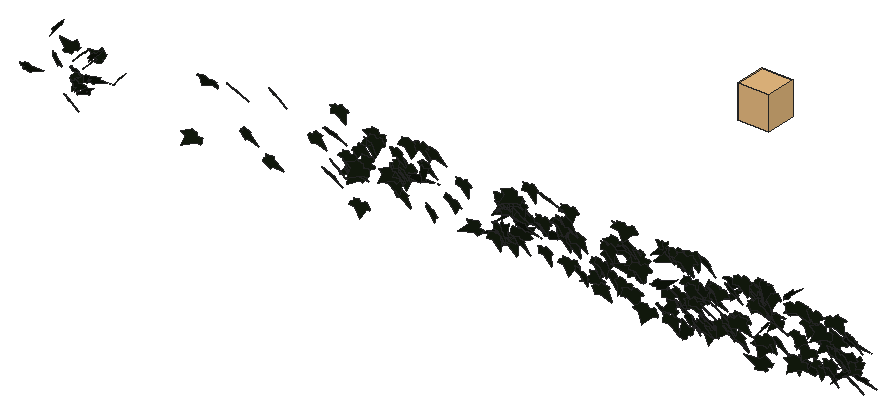
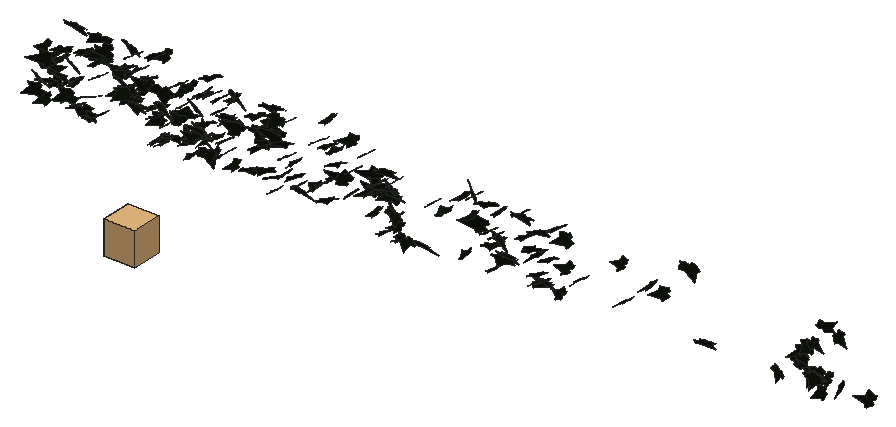
# SketchUp Ruby script. Lengths in millimetres.
U = 1.mm
M = Sketchup.active_model
def pt(a) = Geom::Point3d.new(a.map { |v| v * U })
def face(e, loops, mat)
  f = e.add_face(loops[0].map { |a| pt(a) })
  loops[1..].each { |l| e.add_face(l.map { |a| pt(a) }).erase! }
  f.material = f.back_material = mat if mat
  f
end
# faces: each face lists its corners as indices into pts; further lists are holes
def faces(e, pts, list, mat = nil) = list.each { |f| face(e, (f[0].is_a?(Array) ? f : [f]).map { |l| l.map { |i| pts[i] } }, mat) }
# xy, xz, yz: faces in a plane at the given z, y or x. An outline is a flat list of corners, or four numbers for a rectangle; further outlines are holes
def ring(l) = l.size == 4 ? [[l[0], l[1]], [l[2], l[1]], [l[2], l[3]], [l[0], l[3]]] : l.each_slice(2).to_a
def flat(e, list, mat, &to3) = list.each { |f| face(e, (f[0].is_a?(Array) ? f : [f]).map { |l| ring(l).map { |u, v| to3.(u, v) } }, mat) }
def xy(e, z, list, mat = nil) = flat(e, list, mat) { |x, y| [x, y, z] }
def xz(e, y, list, mat = nil) = flat(e, list, mat) { |x, z| [x, y, z] }
def yz(e, x, list, mat = nil) = flat(e, list, mat) { |y, z| [x, y, z] }
def lines(e, pts, list) = list.each { |a, b| e.add_line(pt(pts[a]), pt(pts[b])) }
# prism: a flat outline (further loops are holes) pulled along v
def prism(e, loops, v, mat = nil)
  f = face(e, loops, mat); d = Geom::Vector3d.new(v.map { |x| x * U })
  f.pushpull(f.normal.samedirection?(d) ? d.length : -d.length)
end
def box(e, o, s, mat = nil) = prism(e, [[o, [o[0] + s[0], o[1], o[2]], [o[0] + s[0], o[1] + s[1], o[2]], [o[0], o[1] + s[1], o[2]]]], [0, 0, s[2]], mat)
def at(x, y, z, deg = 0) = Geom::Transformation.translation(pt([x, y, z])) * Geom::Transformation.rotation(ORIGIN, Z_AXIS, deg.degrees)
def axes(o, x, y, z) = Geom::Transformation.new([*x, 0, *y, 0, *z, 0, *pt(o).to_a, 1])
def part(name) = M.definitions.add(name)
# library, detail: a bought-in or finely detailed component or shape, given as its bounding box
def library(name, o, s) = part(name).tap { |d| box(d.entities, o, s) }
def detail(e, o, s) = box(e.add_group.entities, o, s)
def put(e, d, t, mat = nil) = e.add_instance(d, t).tap { |i| i.material = mat if mat }
def group(e, t, mat = nil) = e.add_group.tap { |g| g.transformation = t; g.material = mat if mat }.entities
root = M.entities
M.materials.add("efeu1").color = [18, 25, 13]
c1 = part("ivyleaf_9")
p = [[39.1,54.8,31.7],[34.5,51.8,30.2],[-5.3,25.2,17.3],[-17.9,28.3,20.9],[-21.6,21.7,17],[-20.2,4.3,5.3],
  [-22.9,-0.3,2.5],[-17.1,-4,-0.6],[-2,-2.1,-1.2],[-0.7,-15.4,-10.1],[16.6,-22.3,-16.7],[21.1,-15.1,-12.5],
  [32.7,-10.7,-11],[46.1,-1.8,-6.6],[30.8,11.2,3.8]]
faces(c1.entities,p,[[0,1,2,3,4,5,6,7,8,9,10,11,12,13,14]],"efeu1")
c2 = library("Spot Light\#3",[-129.6,-129.6,-280.7],[259.2,259.2,280.7])
put(root,c1,axes([27.4,438.3,4934.8],[1.05185,-0.2815,1.21489],[1.46396,-0.21485,-0.90136],[0.41422,1.47415,0.10062]))
put(root,c1,axes([196.1,533.2,5034.4],[1.27663,-0.50201,-0.87336],[-0.8789,0.50729,-1.15475],[0.85903,1.26507,0.11648]))
put(root,c1,axes([300.8,452.1,5346.7],[-0.65532,1.10379,-0.87415],[0.38789,-0.81635,-1.22618],[-1.6734,-0.62148,0.0581]))
put(root,c1,axes([317.8,578.5,4960.4],[1.59905,-0.3934,0.25738],[0.29827,-0.08077,-1.36844],[0.48988,1.33329,-0.00695]))
put(root,c1,axes([454.3,467,4996.8],[-1.46158,-0.32954,-0.68957],[0.90027,-0.16502,-1.20316],[0.2427,-1.37241,0.31025]))
put(root,c1,axes([463.1,479,4983.5],[0.96181,1.16892,0.14934],[0.09715,0.12643,-1.40993],[-1.43439,0.79237,0.00465]))
put(root,c1,axes([507.7,343.1,5276],[0.22927,0.30059,1.46884],[-1.80845,0.25923,0.1366],[-0.27428,-1.45795,0.32713]))
put(root,c1,axes([463,333.7,4901.5],[1.4272,-0.88217,0.28166],[0.28289,-0.16031,-1.46513],[1.09379,1.19254,0.01141]))
put(root,c1,axes([509,407.6,4987.3],[0.93054,0.60119,-1.10895],[-1.1764,-0.55762,-0.96552],[-0.99218,1.22499,0.10473]))
put(root,c1,axes([520.2,565.9,5150.3],[-0.19925,1.30316,-0.58109],[-0.04644,-0.58866,-1.30942],[-1.74013,-0.13351,0.10148]))
put(root,c1,axes([526.5,442.4,5215.2],[-0.8899,1.02361,-0.70913],[0.05509,-0.79955,-1.20058],[-1.51821,-0.629,0.37209]))
put(root,c1,axes([547.3,595.1,5113.7],[-0.56172,0.32471,1.30651],[-1.30957,0.74482,-0.56339],[-0.99127,-1.16799,0.00394]))
put(root,c1,axes([538.7,403.6,4944.4],[0.97215,1.17437,0.25341],[0.14251,0.2269,-1.41887],[-1.45876,0.80479,0.03026]))
put(root,c1,axes([576.3,410.4,5146.4],[0.66606,0.90484,1.05669],[0.25898,1.06766,-1.02392],[-1.67733,0.52415,0.26151]))
put(root,c1,axes([630.5,393.8,5064.3],[1.44137,0.239,0.91451],[1.06503,0.28542,-1.20239],[-0.44218,1.46653,0.08497]))
put(root,c1,axes([694.7,586.7,4995.8],[0.16272,1.21568,0.7693],[-0.05802,0.7759,-1.21787],[-1.75419,0.0871,0.11164]))
put(root,c1,axes([1454.1,460.6,4897.8],[-2.30508,-0.52096,0.19612],[-0.36198,-0.05406,-1.31821],[0.99566,-1.22574,-0.02521]))
put(root,c1,axes([1591.9,413.9,5400.5],[1.5052,0.38712,-1.07511],[-1.91846,-0.37942,-0.87815],[-1.02421,1.2796,0.06487]))
put(root,c1,axes([1620.8,619.3,5265.3],[2.08359,-0.78677,0.26516],[0.48322,-0.10053,-1.34658],[1.50443,1.12194,0.06528]))
put(root,c1,axes([1921.4,392.3,5129.5],[1.44859,-1.06438,-0.49172],[-0.30778,0.48534,-1.30088],[2.21012,0.76522,0.14113]))
put(root,c1,axes([1991.3,606.3,5352.2],[1.37791,-1.03353,0.55169],[0.52453,-0.48009,-1.26106],[2.16713,0.77334,-0.04555]))
put(root,c1,axes([2093.1,420.9,4969.4],[1.52697,-0.79111,-0.80628],[-0.37249,0.87665,-1.05491],[2.1173,0.72477,0.39589]))
put(root,c1,axes([2322.6,627.4,5138.8],[0.76828,-1.09674,-0.68829],[-0.14175,0.7001,-1.15924],[2.46024,0.38282,0.14815]))
put(root,c1,axes([2489.8,642.5,4960.6],[0.75382,-0.95937,0.84674],[0.61245,-0.78321,-1.03792],[2.35706,0.51033,-0.00111]))
put(root,c1,axes([2549.8,599.7,5437.9],[0.01755,-1.33902,-0.38342],[0.03213,0.38351,-1.33892],[2.65065,0.00421,0.01877]))
put(root,c1,axes([2534.6,505.5,5303.9],[2.46874,-0.55053,0.23449],[0.40086,-0.1039,-1.40908],[1.06596,1.31407,-0.01317]))
put(root,c1,axes([2587.1,442.8,5031.7],[1.09046,-1.14178,0.59781],[0.78836,-0.45636,-1.26865],[2.32272,0.69093,0.14994]))
put(root,c1,axes([2668.2,641.4,5011.9],[-2.56331,-0.00456,0.09388],[-0.17862,-0.00694,-1.34683],[0.00958,-1.35009,0.00661]))
put(root,c1,axes([2685.2,634.8,4969.2],[-1.39839,-1.00394,0.51386],[-0.5806,-0.41352,-1.24409],[2.06644,-0.79557,-0.00181]))
put(root,c1,axes([2649.2,634.7,5013.6],[0.60769,-1.07225,-0.76696],[0.3,0.81452,-1.07313],[2.49102,0.16349,0.31634]))
put(root,c1,axes([2675.7,567.9,5134.7],[-0.94128,-1.26783,0.04544],[-0.01331,-0.04605,-1.36085],[2.41445,-0.49452,0.01022]))
put(root,c1,axes([2708.9,611,5186.2],[0.81813,-0.73139,-1.07949],[-0.45428,1.0733,-0.82225],[2.43971,0.44511,0.20889]))
put(root,c1,axes([2853.7,556.1,5138.9],[-1.39855,-0.28673,1.11502],[-1.8365,-0.56812,-0.78203],[1.19515,-1.20851,0.10308]))
put(root,c1,axes([2830.1,608.1,5275.6],[-0.51347,-1.3436,-0.18841],[0.02425,0.18958,-1.3702],[2.58204,-0.26897,-0.0246]))
put(root,c1,axes([2872.4,435.9,4898.2],[-0.87636,-1.26984,-0.02353],[-0.01503,0.02789,-1.35064],[2.41712,-0.46022,-0.01693]))
put(root,c1,axes([2904.4,402.6,5191.3],[-2.02144,-0.92998,0.44622],[-0.58815,-0.32417,-1.4112],[1.87296,-1.1055,0.03845]))
put(root,c1,axes([2914.8,560.2,5383],[-2.49156,-0.45963,-0.17804],[0.30501,0.08089,-1.38729],[0.88713,-1.31872,-0.02305]))
put(root,c1,axes([2937.6,517.9,5369.9],[-0.40079,-1.3596,0.21791],[-0.11885,-0.21078,-1.3755],[2.61792,-0.21772,-0.02909]))
put(root,c1,axes([3000.1,617.9,5083.2],[-2.58496,-0.18615,0.01166],[-0.00965,-0.04877,-1.37009],[0.35484,-1.35739,0.04763]))
put(root,c1,axes([3002.3,615.5,5051.4],[-1.51928,-0.58379,-0.95076],[1.4529,0.56673,-0.98896],[1.54848,-1.10454,-0.00491]))
put(root,c1,axes([3063.2,601.3,5191.8],[-0.82913,1.30172,0.21151],[-0.1436,0.19778,-1.37266],[-2.50581,-0.44205,0.00868]))
put(root,c1,axes([3029.9,607.7,5155.3],[0.79861,-1.30874,0.10938],[0.04056,-0.10802,-1.37431],[2.49915,0.41996,-0.01265]))
put(root,c1,axes([3050.7,625.1,4964.6],[0.76216,-1.2942,-0.11492],[0.14171,0.14291,-1.35003],[2.46876,0.39135,0.11297]))
put(root,c1,axes([3067.2,604.7,5198],[0.28453,-1.3587,-0.23646],[-0.00235,0.23772,-1.36669],[2.62475,0.1475,0.02441]))
put(root,c1,axes([3107.6,611.9,5120.5],[-1.01144,-1.22449,-0.33365],[0.1904,0.32018,-1.3344],[2.4079,-0.53966,-0.03464]))
put(root,c1,axes([3090.7,529.2,5335.7],[0.94962,-1.29655,-0.07612],[-0.03525,0.07443,-1.38921],[2.47158,0.49921,0.00943]))
put(root,c1,axes([3135.9,604,5204.8],[-0.34265,-1.37168,0.08],[0.01061,-0.08141,-1.38335],[2.61499,-0.1794,0.01609]))
put(root,c1,axes([3172.3,591.3,5398.3],[-1.26405,-1.19263,-0.35048],[0.56016,0.23519,-1.35808],[2.29853,-0.71319,0.13823]))
put(root,c1,axes([3235.2,539.9,5179.2],[1.75515,-0.22884,1.07308],[2.06405,-0.02249,-0.93683],[0.31672,1.41473,0.15868]))
put(root,c1,axes([3269.2,579.1,5416.7],[0.42641,-1.38648,-0.15003],[0.03127,0.15456,-1.40388],[2.65397,0.22094,0.04064]))
put(root,c1,axes([3270.7,596.1,5270.7],[1.39207,-1.16552,-0.24444],[-0.01661,0.28161,-1.36887],[2.26642,0.71794,0.14011]))
put(root,c1,axes([3338.9,593.4,4944.2],[0.21321,-1.0973,0.79828],[0.13508,-0.79516,-1.10297],[2.57901,0.13236,-0.00822]))
put(root,c1,axes([3343.1,586.3,5393],[1.50238,-1.09313,-0.41091],[-0.02661,0.4871,-1.32267],[2.22241,0.7448,0.26195]))
put(root,c1,axes([3389.8,435.3,5286.3],[-0.32853,0.80836,1.24038],[0.05217,-1.24682,0.81637],[2.81727,0.11735,0.12953]))
put(root,c1,axes([3588.2,510.7,5142.5],[-0.24682,-1.22769,0.81297],[0.46358,-0.82276,-1.20362],[2.76378,0.02836,0.27449]))
put(root,c1,axes([3608.9,596.2,5251.1],[0.18815,-1.39101,0.07323],[-0.0011,-0.07346,-1.3945],[2.65103,0.09869,-0.00577]))
put(root,c1,axes([3705.6,631.8,4922.3],[-2.4814,0.23628,0.28342],[-0.54889,-0.00331,-1.32396],[-0.43807,-1.33425,0.05348]))
put(root,c1,axes([3805.9,638.6,4928.4],[0.91824,1.23788,0.21388],[0.02256,0.22461,-1.32676],[-2.39074,0.47757,0.06963]))
put(root,c1,axes([3849.2,642.7,4911.6],[-0.2939,-1.31308,-0.17275],[0.14815,0.16462,-1.32087],[2.51622,-0.16306,0.05759]))
put(root,c1,axes([3862.8,632.5,4988.7],[1.36079,-1.12468,0.2344],[0.32497,-0.16899,-1.33168],[2.1622,0.73322,0.05263]))
put(root,c1,axes([3920.2,624.3,5069.5],[0.39316,1.23635,0.53611],[-0.08804,0.54856,-1.24723],[-2.5632,0.1708,0.12507]))
put(root,c1,axes([3922.9,588,5025.8],[0.32018,-1.32871,0.17319],[-0.01074,-0.17525,-1.33904],[2.55017,0.16609,-0.02738]))
put(root,c1,axes([3948.6,651.9,4942.2],[-1.40473,-1.01334,0.44205],[0.04449,-0.5457,-1.2119],[2.10363,-0.66513,0.32081]))
put(root,c1,axes([3992.8,604.5,5185],[-2.42646,-0.41448,0.3082],[-0.55089,-0.10647,-1.34057],[0.81415,-1.30733,0.01146]))
put(root,c1,axes([3947.3,569.6,5282.4],[0.62887,-1.30908,-0.36857],[-0.15548,0.3595,-1.35011],[2.58363,0.34027,0.00846]))
put(root,c1,axes([3946,570.6,5167.4],[1.69821,0.56573,0.94393],[1.36699,0.62131,-1.05134],[-1.58681,1.14068,0.1045]))
put(root,c1,axes([3992.1,588,5240.8],[-1.91952,0.60212,-0.72264],[1.09829,-0.4406,-1.17253],[-1.41368,-1.15987,0.07027]))
put(root,c1,axes([3982.5,556,5018.4],[-0.59803,0.76039,1.16127],[0.16815,-1.17728,0.79478],[2.63642,0.24757,0.21272]))
put(root,c1,axes([3978.5,637.2,4922.8],[-0.0552,-1.31423,-0.28767],[0.09639,0.28647,-1.31383],[2.55864,-0.03914,0.04329]))
put(root,c1,axes([3992.6,598.1,5197.2],[0.17116,-1.21194,-0.83529],[0.04314,0.83789,-1.21327],[2.801,0.06115,0.06973]))
put(root,c1,axes([4071.4,571.1,5317.9],[-2.32749,-0.57852,0.32969],[-0.57435,-0.13302,-1.35284],[1.12965,-1.25959,-0.00855]))
put(root,c1,axes([4039.4,614.6,5260.5],[0.98796,-1.22683,-0.33742],[0.1792,0.40046,-1.31118],[2.41497,0.47218,0.23533]))
put(root,c1,axes([4052.6,604.8,5247.8],[-1.33794,-0.31713,-1.14848],[1.95784,0.5112,-0.77084],[1.14402,-1.24574,-0.02396]))
put(root,c1,axes([4112.5,608,5155.2],[-0.4617,-1.32443,0.16967],[-0.03587,-0.16903,-1.34642],[2.54101,-0.24304,0.01182]))
put(root,c1,axes([4099,571.4,4996.7],[1.29671,-1.17117,-0.11113],[-0.08725,0.10189,-1.35489],[2.23728,0.68277,0.01157]))
put(root,c1,axes([4124.9,625.9,5160.2],[1.58313,-1.04884,-0.25108],[0.06039,0.34075,-1.3183],[2.05166,0.79929,0.23255]))
put(root,c1,axes([4164.4,498.8,5079.9],[-0.90224,-0.12342,1.36757],[2.60771,0.05229,0.47969],[-0.17124,1.44646,0.09935]))
put(root,c1,axes([4179.5,588.1,5418.9],[0.11544,-1.40388,-0.04886],[-0.00007,0.04891,-1.40519],[2.67349,0.06062,0.00207]))
put(root,c1,axes([4183.9,466.9,5184],[1.90871,-0.63853,0.94186],[1.47476,-0.53615,-1.18858],[1.58592,1.26706,-0.0283]))
put(root,c1,axes([4316.5,555.2,5232.5],[-0.00652,-1.39002,0.04837],[-0.0068,-0.04836,-1.39002],[2.64707,-0.00355,-0.00345]))
put(root,c1,axes([4349.8,528.2,5026.8],[0.54484,-1.37135,0.00656],[-0.03134,-0.01014,-1.40079],[2.60979,0.28617,-0.01819]))
put(root,c1,axes([4334.8,530.6,5430.9],[1.87033,-0.96991,0.26855],[0.75541,0.02861,-1.34916],[1.76012,1.01836,0.29367]))
put(root,c1,axes([4381.8,555.5,5127.5],[0.60322,-0.26386,1.3366],[2.54975,0.30972,-0.25654],[-0.47116,1.3383,0.3229]))
put(root,c1,axes([4454.3,594.4,5244.8],[-1.09471,-1.23427,0.15405],[-0.07881,-0.15062,-1.36147],[2.36598,-0.5761,0.02592]))
put(root,c1,axes([4451.6,596.3,5137.9],[0.62324,-1.30622,0.20665],[0.08227,-0.2022,-1.34663],[2.51558,0.33023,-0.00716]))
put(root,c1,axes([4511.8,600.6,4960.6],[-1.02138,-1.23264,-0.08332],[0.04287,0.08107,-1.34435],[2.35093,-0.53701,-0.01169]))
put(root,c1,axes([4511.2,590.8,5365.7],[-0.53481,-1.36172,-0.12119],[0.01589,0.12202,-1.39032],[2.60182,-0.28065,-0.01642]))
put(root,c1,axes([4507.7,626.6,5100.3],[0.43667,-1.32212,-0.17693],[-0.00742,0.17887,-1.34162],[2.53868,0.22793,0.02651]))
put(root,c1,axes([4514.4,508.9,5279.5],[-0.47991,-1.15811,0.72503],[0.4045,-0.76155,-1.14252],[2.56877,-0.09644,0.31536]))
put(root,c1,axes([4651.8,374.2,5422.5],[1.27655,-1.24246,-0.16385],[-0.09675,0.15872,-1.41162],[2.38315,0.67198,0.03046]))
put(root,c2,at(4685.4,2446,5575.8))
put(root,c1,axes([4660.9,530.6,4963.1],[0.32459,-1.19124,0.68306],[0.37896,-0.65957,-1.20001],[2.58582,0.2462,0.09013]))
put(root,c1,axes([4681.7,442.8,5281.4],[0.54619,-1.30151,-0.45817],[0.20835,0.48798,-1.31761],[2.61775,0.23272,0.20047]))
put(root,c1,axes([4717.8,638,5008.7],[-0.22003,-1.28429,0.3593],[-0.061,-0.35786,-1.28948],[2.53738,-0.11997,0.00015]))
put(root,c1,axes([4781.9,576.7,4933.7],[-2.45904,0.33889,0.37968],[-0.69924,0.09577,-1.33576],[-0.67024,-1.34327,0.00055]))
put(root,c1,axes([4834.8,537.6,5090.5],[0.05065,-1.34022,0.46195],[0.112,-0.46059,-1.33966],[2.69565,0.04432,0.04698]))
put(root,c1,axes([4874.8,578.2,5142.7],[-0.5591,-1.25064,0.52529],[-0.0267,-0.53463,-1.28074],[2.58151,-0.27639,0.10052]))
put(root,c1,axes([4870,465.3,4955],[0.37142,-1.16352,-0.71686],[0.10063,0.73002,-1.17048],[2.59902,0.13801,0.14776]))
put(root,c1,axes([4876,576.9,5012.4],[0.30461,-1.33128,0.18881],[-0.01479,-0.19105,-1.34053],[2.55901,0.15736,-0.03022]))
put(root,c1,axes([4910.2,605.4,5247],[-1.63388,-1.07382,0.14791],[-0.08686,-0.15271,-1.37352],[2.06116,-0.85765,0.05937]))
put(root,c1,axes([4902.6,655.8,4914.2],[-0.03545,-1.30347,0.24935],[0.07923,-0.24983,-1.30285],[2.52451,-0.01046,0.04439]))
put(root,c1,axes([4947.5,563.3,5405.7],[2.53486,-0.02046,-0.50214],[-0.93409,0.25288,-1.31212],[0.20566,1.40076,0.22954]))
put(root,c1,axes([4985.1,596.5,4960.1],[-1.35112,-1.06443,0.44559],[-0.19285,-0.46364,-1.26898],[2.18769,-0.69826,0.16333]))
put(root,c1,axes([4970.8,429.2,5314.5],[0.08297,-1.41863,0.05695],[0.00847,-0.05684,-1.4193],[2.7021,0.04374,0.0027]))
put(root,c1,axes([4974.8,526.7,5236.1],[0.9889,-0.16158,1.32532],[2.52249,0.23386,-0.49112],[-0.30631,1.40419,0.2343]))
put(root,c1,axes([5049.9,522.4,5445],[-1.97504,-0.88039,-0.44682],[0.73167,0.23674,-1.35934],[1.73069,-1.10477,0.06478]))
put(root,c1,axes([5120.5,534,5130.7],[-1.24429,0.04671,1.2732],[-2.40277,-0.21614,-0.64036],[0.32598,-1.41484,0.13986]))
put(root,c1,axes([5054.6,536.8,5268.4],[-1.57251,-0.6682,-0.95212],[1.37631,0.61967,-1.06243],[1.73397,-1.09783,-0.02017]))
put(root,c1,axes([5045.4,526.7,5327.5],[0.78938,-1.29731,0.38748],[0.21971,-0.36989,-1.362],[2.56743,0.43052,-0.00258]))
put(root,c1,axes([5080.1,538.7,4962.8],[-0.6423,-1.1931,-0.69454],[0.4314,0.6574,-1.23944],[2.59178,-0.4051,0.03418]))
put(root,c1,axes([5099.1,583.5,5142.1],[-0.19426,-1.26752,-0.5716],[0.08236,0.56997,-1.27162],[2.64501,-0.11084,-0.00239]))
put(root,c1,axes([5118.1,546.8,5253.6],[-0.77217,-1.16314,0.63076],[-0.13732,-0.63932,-1.22533],[2.51449,-0.3921,0.12678]))
put(root,c1,axes([5173.1,542.9,5244.8],[-2.22555,-0.64385,0.53498],[-0.88105,-0.26836,-1.33486],[1.32738,-1.25762,0.01095]))
put(root,c1,axes([5140.9,506.5,5125.6],[-0.18837,0.18185,1.45176],[0.61529,-1.4164,0.19946],[2.71576,0.33352,0.05551]))
put(root,c1,axes([5240.3,513.1,4895.5],[-1.64311,-1.22428,0.02958],[-0.02012,-0.02874,-1.49805],[2.33064,-0.86337,0.00792]))
put(root,c1,axes([5252.9,420.5,5262.5],[-0.87358,-1.28293,-0.40304],[0.23447,0.38397,-1.36251],[2.54856,-0.47508,-0.0128]))
put(root,c1,axes([5370.8,618.7,5296.6],[-2.32489,-0.39612,0.48577],[-0.87902,-0.15052,-1.28419],[0.80649,-1.30597,0.00067]))
put(root,c1,axes([5305.9,553.6,4920.8],[1.67246,-1.00952,-0.04734],[-0.0527,0.03866,-1.33841],[1.92271,0.87919,0.00449]))
put(root,c1,axes([5386.2,502.7,5412],[-1.81271,1.0759,-0.2968],[0.39163,-0.21422,-1.43686],[-2.08772,-0.97436,-0.01183]))
put(root,c1,axes([5331.7,542.8,5407.4],[1.09857,-1.29926,0.06332],[0.04553,-0.05866,-1.42171],[2.47527,0.57772,-0.00195]))
put(root,c1,axes([5344,590.4,5026.4],[0.43561,-1.3565,-0.16098],[-0.00324,0.16294,-1.37544],[2.5998,0.22749,0.02526]))
put(root,c1,axes([5356.7,472.1,5129.9],[0.21841,-0.21163,1.43679],[2.60562,0.49664,-0.0362],[-0.92219,1.3531,0.238]))
put(root,c1,axes([5408.4,609.4,5320.6],[0.12918,-1.36175,-0.14946],[-0.01656,0.14921,-1.36344],[2.6072,0.06842,-0.00126]))
put(root,c1,axes([5442.9,559.7,5384.1],[0.2021,-1.39244,-0.29469],[-0.06503,0.29293,-1.39643],[2.708,0.11095,-0.01154]))
put(root,c1,axes([5503.8,605.4,4971.5],[0.72072,1.19675,-0.49344],[-0.40955,-0.44877,-1.25355],[-2.42938,0.43069,0.06494]))
put(root,c1,axes([5470.4,571.2,5070.8],[-0.3233,-1.19487,0.69858],[0.25429,-0.71469,-1.18994],[2.62191,-0.07802,0.20155]))
put(root,c1,axes([5459.8,589.2,4962.7],[0.8269,-1.13903,0.66149],[0.43157,-0.62146,-1.21905],[2.46941,0.49002,-0.00845]))
put(root,c1,axes([5514.9,408.3,4975.7],[0.1594,-1.39141,-0.30198],[0.03707,0.30359,-1.39344],[2.70953,0.0777,0.03683]))
put(root,c1,axes([5543.8,599.2,5174],[-0.82651,-1.31166,-0.15494],[0.0626,0.15231,-1.38159],[2.51294,-0.4352,-0.01654]))
put(root,c1,axes([5568.6,382.5,5072.6],[-0.86568,-0.48635,1.32151],[-1.22082,-1.16472,-0.64944],[2.38581,-0.77246,0.14718]))
put(root,c1,axes([5535.5,516.5,5365.5],[0.39181,-1.34072,-0.43835],[0.13761,0.45244,-1.34986],[2.68105,0.17271,0.13334]))
put(root,c1,axes([5559.2,586.4,5386.3],[-0.22815,-1.35425,-0.37068],[0.17765,0.36352,-1.35827],[2.6663,-0.1401,0.05878]))
put(root,c1,axes([5563.3,567.2,5048.7],[0.62951,-1.22251,-0.58126],[0.08175,0.60754,-1.25334],[2.57498,0.27958,0.18189]))
put(root,c1,axes([5647.5,420.5,4884.2],[-2.11658,0.5975,-0.80749],[-1.40059,0.33534,1.26168],[1.30126,1.33281,0.04455]))
put(root,c1,axes([5651,596.5,5103.5],[-2.5867,-0.13324,-0.0068],[0.01447,-0.00781,-1.36562],[0.25349,-1.35913,0.00851]))
put(root,c1,axes([5610.7,455.9,5440.4],[-0.86518,-1.33089,-0.26563],[0.23182,0.23899,-1.40589],[2.57249,-0.46914,0.03736]))
put(root,c1,axes([5663.2,541.1,5090.7],[-2.27219,0.63723,0.09578],[-0.17207,0.03402,-1.35324],[-1.21427,-1.19723,0.01253]))
put(root,c1,axes([5607.7,478.3,4983.3],[1.66794,-1.01627,-0.57294],[-0.70083,0.439,-1.34194],[2.10686,0.95058,0.0072]))
put(root,c1,axes([5645.3,611.3,4892.3],[0.08092,-1.26087,0.50961],[0.21461,-0.50483,-1.25846],[2.57937,0.08156,0.08872]))
put(root,c1,axes([5628.5,590.2,5017.3],[0.95994,-0.88301,0.95682],[1.02353,-0.79319,-1.0155],[2.25671,0.73536,0.05357]))
put(root,c1,axes([5736.4,468.5,5182.3],[-1.83032,0.65482,-0.93734],[-1.4502,0.54618,1.16334],[1.62251,1.22686,-0.01761]))
put(root,c1,axes([5669.1,567.8,5389.5],[1.17535,-1.22369,0.35614],[0.26599,-0.32834,-1.37052],[2.41094,0.63279,-0.02242]))
put(root,c1,axes([5693.6,376.9,5273.7],[1.52755,-0.82109,-0.89977],[-0.55215,0.91767,-1.09621],[2.25157,0.78209,0.34161]))
put(root,c1,axes([5744.8,550.9,5144.3],[-2.4183,-0.26749,0.60784],[1.15388,0.06827,1.29744],[-0.51578,1.4069,0.05261]))
put(root,c1,axes([5701.1,418.6,5009.8],[0.40697,-0.0716,-1.40799],[2.46126,-0.55709,0.22473],[-1.06838,-1.31065,-0.01861]))
put(root,c1,axes([5711.1,545.5,4959.5],[-0.57198,-0.45039,1.24694],[0.98324,-1.21729,-0.31516],[2.32377,0.4042,0.44027]))
put(root,c1,axes([5726.6,440.5,4987.9],[1.67065,-0.99672,-0.47626],[-0.34152,0.47159,-1.31766],[2.07447,0.88033,0.16663]))
put(root,c1,axes([5766.4,516,4912.2],[-0.7792,-1.2876,0.23439],[-0.10333,-0.22867,-1.35101],[2.48869,-0.41264,0.01729]))
put(root,c1,axes([5767.1,579.2,5210.9],[-0.38405,-1.3009,0.4104],[-0.20656,-0.39824,-1.31572],[2.58793,-0.22484,-0.04411]))
put(root,c1,axes([5788,546,5080.9],[0.44324,-0.9554,1.01097],[0.94745,-0.8999,-0.96512],[2.47199,0.51622,0.18863]))
put(root,c1,axes([5849,574.5,4955.6],[-2.0184,-0.84527,-0.02285],[0.1447,-0.05881,-1.35296],[1.60279,-1.05914,0.09337]))
put(root,c1,axes([5911.7,616.6,5191.7],[-1.37141,1.16773,-0.10601],[-0.05094,-0.14078,-1.36877],[-2.23098,-0.7146,0.09642]))
put(root,c1,axes([5850.6,433.4,5237.9],[1.90578,-0.86999,-0.55666],[-0.51338,0.52813,-1.31064],[1.89748,1.01669,0.20449]))
put(root,c1,axes([5849.7,602.4,4936.3],[1.32978,-1.09307,-0.48421],[-0.14465,0.51909,-1.28149],[2.27071,0.67319,0.20193]))
put(root,c1,axes([5905.7,597.5,5304],[1.74037,0.51736,-0.92018],[-1.54929,-0.4295,-1.05045],[-1.27913,1.22412,0.02033]))
put(root,c1,axes([5882.7,469.9,5284.8],[-0.77262,-1.27659,0.53916],[0.12135,-0.57843,-1.32156],[2.63462,-0.34773,0.21898]))
put(root,c1,axes([5885.5,553.3,5031.4],[0.42744,-1.36089,-0.08072],[0.00535,0.08227,-1.3792],[2.59459,0.22403,0.01614]))
put(root,c1,axes([5905.1,562.9,4922.1],[1.80198,-0.90171,-0.3328],[-0.15036,0.39257,-1.28839],[1.82309,0.92364,0.22269]))
put(root,c1,axes([5934.6,593.5,4908.5],[1.0399,-1.32625,-0.23181],[-0.13652,0.22114,-1.43429],[2.55875,0.5508,0.01768]))
put(root,c1,axes([5938.2,558.2,5054.2],[2.42744,-0.59538,-0.15496],[-0.24989,0.08505,-1.40741],[1.14391,1.28201,0.0214]))
put(root,c1,axes([5981.2,582.2,5066],[-0.88049,-1.28753,0.21412],[-0.07329,-0.21361,-1.36766],[2.483,-0.46287,0.03556]))
put(root,c1,axes([6007.5,485.4,5095.2],[0.41834,-1.15176,-0.93886],[0.33079,0.96249,-1.14006],[2.80862,0.05819,0.27411]))
put(root,c1,axes([6026.8,597.6,5271.3],[-0.12207,-0.42074,1.32367],[2.54946,0.3314,0.17024],[-0.69848,1.28312,0.39006]))
put(root,c1,axes([6046,572.2,5331.3],[-0.29983,-1.35733,-0.37921],[0.33934,0.35931,-1.36017],[2.66064,-0.19879,0.13075]))
put(root,c1,axes([6039.1,364.3,5408.9],[1.75433,-1.13065,0.0773],[0.05643,-0.07555,-1.45857],[2.15614,0.92193,-0.02472]))
put(root,c1,axes([6067.9,579.8,5303.3],[1.78136,-0.96297,-0.44928],[-0.22941,0.49863,-1.31987],[2.00933,0.91065,0.24761]))
put(root,c1,axes([6081.8,452.8,5442.8],[-0.09099,-1.41611,-0.37192],[-0.0309,0.37261,-1.41665],[2.78638,-0.04211,-0.02785]))
put(root,c1,axes([6086.9,568.2,5205.8],[0.90703,-0.87766,-1.00415],[-0.12761,1.04922,-0.94888],[2.53498,0.36685,0.31152]))
put(root,c1,axes([6187,601.5,5175.1],[2.6378,0.09916,-0.0159],[-0.08248,0.39206,-1.33246],[-0.17241,1.32947,0.39413]))
put(root,c1,axes([6191,462.7,5300.1],[0.65774,-1.27743,-0.64256],[0.06824,0.6686,-1.3099],[2.72059,0.29207,0.1882]))
put(root,c1,axes([6217.1,527.8,5418],[-0.67126,-1.27966,0.46207],[-0.08037,-0.46682,-1.32505],[2.58812,-0.34639,0.0787]))
put(root,c1,axes([6213.8,521.5,5282.3],[0.73246,-1.33659,0.25682],[0.07267,-0.25618,-1.39048],[2.5893,0.38528,-0.03363]))
put(root,c1,axes([6255.1,501.8,5136.3],[-1.08077,0.55902,-1.13845],[1.05111,-1.01388,-0.77335],[-2.17294,-0.76849,0.19215]))
put(root,c1,axes([6242.5,567.6,5337],[-0.73083,-1.37574,0.05416],[0.00522,-0.057,-1.42822],[2.62034,-0.38359,0.01795]))
put(root,c1,axes([6261.6,462.4,5006.9],[-2.39381,-0.15183,-0.71672],[1.34234,0.13426,-1.2662],[0.37718,-1.44141,-0.04244]))
put(root,c1,axes([6279.8,474.2,5451.2],[-2.13928,0.08151,-0.97216],[1.84655,-0.0615,-1.12698],[-0.19391,-1.48485,-0.00669]))
put(root,c1,axes([6256.9,464.6,5054.3],[-0.28656,-0.99929,-1.02047],[0.79374,0.95064,-0.99245],[2.59981,-0.40038,0.19052]))
put(root,c1,axes([6361.5,354.1,4923.9],[-0.79283,0.42238,1.24961],[-2.24923,0.46251,-0.55031],[-1.115,-1.23334,0.22158]))
put(root,c1,axes([6344.5,517.2,5196],[-2.41929,0.33638,-0.48656],[0.91367,-0.08711,-1.31443],[-0.65773,-1.35832,-0.0362]))
put(root,c1,axes([6346.1,459.3,5201.4],[0.81088,-0.96732,1.05916],[1.17533,-0.87355,-1.04622],[2.46399,0.73502,0.15049]))
put(root,c1,axes([6363.5,469.7,5070.4],[1.63938,-1.14204,-0.12492],[-0.12122,0.10842,-1.43039],[2.18314,0.86361,0.01438]))
put(root,c1,axes([6398.5,537.3,5386.9],[0.72696,0.29617,1.38633],[1.63678,1.09297,-0.47045],[-2.1448,0.93447,0.11087]))
put(root,c1,axes([6447.4,572.4,4913.6],[-0.17938,-1.39177,0.02875],[0.00885,-0.02913,-1.39495],[2.64937,-0.09413,0.00661]))
put(root,c1,axes([6456.1,565.2,5308.2],[1.13458,-1.26435,-0.1792],[-0.06759,0.18127,-1.39712],[2.42941,0.59552,0.04482]))
put(root,c1,axes([6469,477.4,5314.1],[2.19294,0.21532,0.78492],[1.34311,0.41349,-1.1494],[-0.77174,1.33146,0.23001]))
put(root,c1,axes([6526.6,510.7,5140.6],[-0.75567,-1.23988,0.48188],[-0.16119,-0.4783,-1.30046],[2.52655,-0.40135,0.06116]))
put(root,c1,axes([6544.4,583.2,5014.8],[-1.5485,-1.05901,0.39058],[0.12928,-0.52654,-1.28615],[2.14432,-0.73301,0.35959]))
put(root,c1,axes([6581,584.4,4918.1],[-0.36604,1.0084,-0.84269],[-0.12581,-0.85801,-1.01165],[-2.49792,-0.10455,0.17444]))
put(root,c1,axes([6600.5,579.2,4867.8],[0.00168,-0.02103,1.42557],[-1.71533,1.10458,0.01685],[-2.10248,-0.9012,-0.01261]))
put(root,c1,axes([6541.9,442.8,5409.2],[-0.64032,-0.73611,-1.20925],[1.45089,0.95312,-0.7923],[2.2703,-0.81673,0.16528]))
put(root,c1,axes([6609.9,546.8,5330.3],[-0.56748,-1.34633,-0.23267],[0.06414,0.23083,-1.37885],[2.59953,-0.2996,-0.01677]))
put(root,c1,axes([6598.4,612.7,5126.1],[1.15225,-1.21547,-0.14231],[-0.09167,0.13498,-1.3578],[2.32727,0.60711,0.01698]))
put(root,c1,axes([6644.3,496.9,5276.8],[-1.05289,-1.27362,0.34792],[-0.18995,-0.33581,-1.38798],[2.50558,-0.56066,0.04098]))
put(root,c1,axes([6641.4,597.9,4924.8],[-0.63301,-1.3287,0.08853],[-0.0194,-0.08871,-1.36965],[2.53432,-0.33256,0.01163]))
put(root,c1,axes([6674.2,622.1,5110.4],[-0.286,-1.34797,-0.16312],[0.02471,0.16268,-1.35631],[2.58405,-0.15075,-0.00508]))
put(root,c1,axes([6715.6,273.8,5113.5],[-2.3939,-0.66564,0.04181],[-0.06868,-0.02119,-1.4231],[1.26749,-1.25835,0.00185]))
put(root,c1,axes([6702.2,558.3,4956.5],[1.99327,0.51327,0.70659],[1.11745,0.40294,-1.16298],[-1.23045,1.19741,0.08847]))
put(root,c1,axes([6783.1,617.9,5117.6],[-2.64203,0.25948,-0.4971],[-0.95031,0.03201,1.4111],[0.48568,1.47417,0.05686]))
put(root,c1,axes([6781.8,497.6,5176.6],[-2.32011,0.53589,-0.45467],[0.80145,-0.17183,-1.33159],[-1.07082,-1.28969,-0.01151]))
put(root,c1,axes([6731.8,557.3,4931.6],[0.93815,-1.27615,0.10835],[0.0433,-0.10736,-1.36793],[2.43712,0.49315,-0.01741]))
put(root,c1,axes([6753.3,591.4,5315.2],[-0.22642,-1.14962,-0.94907],[0.16342,0.94523,-1.15572],[2.8325,-0.14643,-0.00919]))
put(root,c1,axes([6768,520.6,5022.8],[0.48716,-1.34178,-0.05555],[-0.03304,0.05324,-1.36596],[2.55565,0.25646,-0.00707]))
put(root,c1,axes([6864,355.6,5359.9],[-2.78332,-0.17997,-0.09726],[0.18378,0.0116,-1.47347],[0.34322,-1.46562,0.00028]))
put(root,c1,axes([6912.3,543.8,5080.1],[0.37684,-0.141,1.37987],[-2.25465,0.70779,0.24232],[-1.37305,-1.20094,-0.01919]))
put(root,c1,axes([6839.3,477.7,5151.9],[0.74832,-1.37533,0.27106],[0.14584,-0.26001,-1.43043],[2.66388,0.40058,0.00217]))
put(root,c1,axes([6896.4,503.1,4991.7],[-0.44439,0.83704,-1.05981],[0.42654,-1.03661,-0.86809],[-2.53463,-0.3212,0.03973]))
put(root,c1,axes([6865.6,601.3,4900.2],[2.02833,-0.85983,-0.0985],[-0.13981,0.06581,-1.36935],[1.64119,1.06827,0.00508]))
put(root,c1,axes([6924.2,590.5,5016.9],[-2.06981,-0.82835,0.23481],[-0.09302,-0.31829,-1.34921],[1.636,-1.0661,0.22037]))
put(root,c1,axes([6863.3,591.3,5189.4],[2.25896,-0.31127,0.79352],[1.44344,-0.23523,-1.22671],[0.74041,1.40824,-0.02951]))
put(root,c1,axes([6961.5,609.8,5047.1],[-2.18961,0.45272,-0.54823],[0.82246,-0.38285,-1.22304],[-1.07453,-1.21557,0.18102]))
put(root,c1,axes([6911.8,464,5144.4],[0.71937,-1.26334,0.48366],[0.28383,-0.46021,-1.31864],[2.55888,0.4062,0.01029]))
put(root,c1,axes([6916.2,554.5,5250.3],[1.21926,-1.21051,0.35995],[0.31769,-0.31891,-1.36958],[2.38245,0.66202,-0.00158]))
put(root,c1,axes([6943.5,599.1,4941.4],[2.46358,-0.24286,0.25292],[0.46158,-0.07849,-1.31664],[0.48196,1.31658,-0.03184]))
